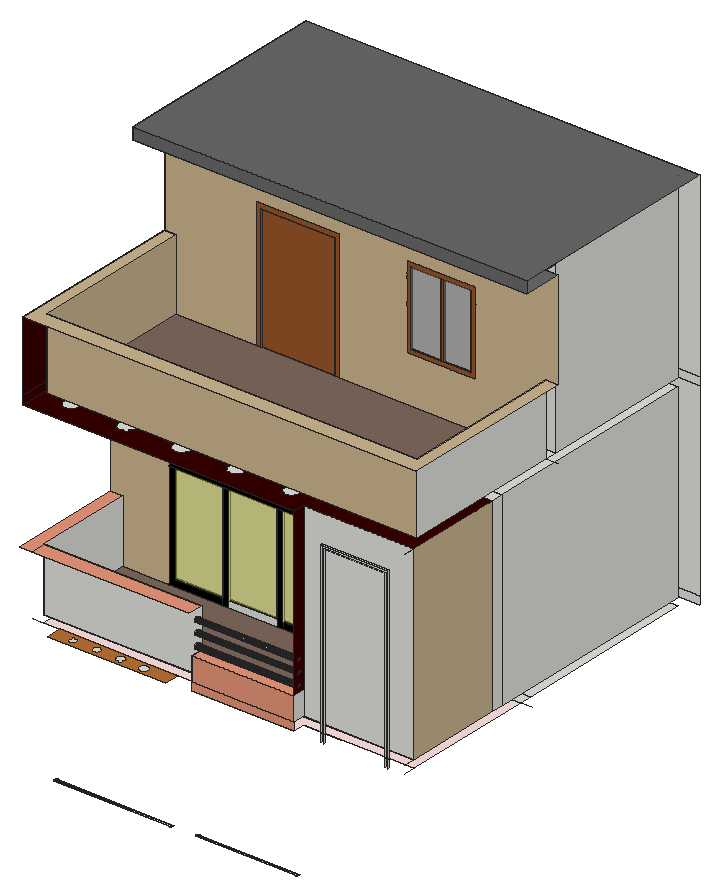
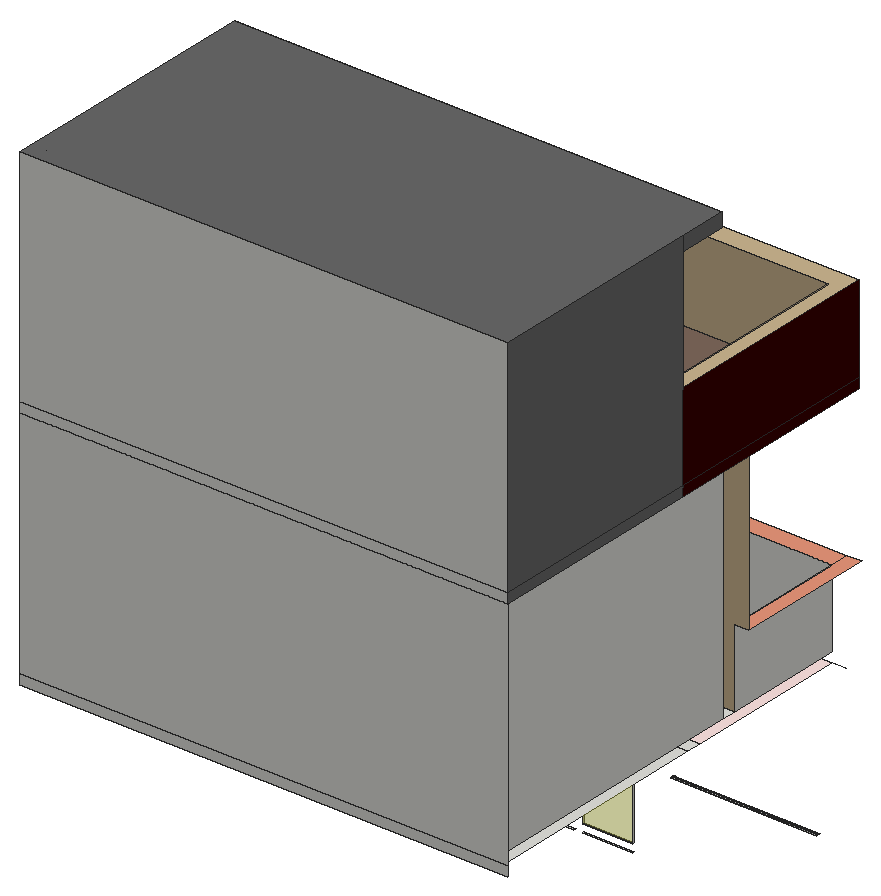
# SketchUp Ruby script. Lengths in inches.
U = 1.inch
M = Sketchup.active_model
def pt(a) = Geom::Point3d.new(a.map { |v| v * U })
def face(e, loops, mat)
  f = e.add_face(loops[0].map { |a| pt(a) })
  loops[1..].each { |l| e.add_face(l.map { |a| pt(a) }).erase! }
  f.material = f.back_material = mat if mat
  f
end
# faces: each face lists its corners as indices into pts; further lists are holes
def faces(e, pts, list, mat = nil) = list.each { |f| face(e, (f[0].is_a?(Array) ? f : [f]).map { |l| l.map { |i| pts[i] } }, mat) }
# xy, xz, yz: faces in a plane at the given z, y or x. An outline is a flat list of corners, or four numbers for a rectangle; further outlines are holes
def ring(l) = l.size == 4 ? [[l[0], l[1]], [l[2], l[1]], [l[2], l[3]], [l[0], l[3]]] : l.each_slice(2).to_a
def flat(e, list, mat, &to3) = list.each { |f| face(e, (f[0].is_a?(Array) ? f : [f]).map { |l| ring(l).map { |u, v| to3.(u, v) } }, mat) }
def xy(e, z, list, mat = nil) = flat(e, list, mat) { |x, y| [x, y, z] }
def xz(e, y, list, mat = nil) = flat(e, list, mat) { |x, z| [x, y, z] }
def yz(e, x, list, mat = nil) = flat(e, list, mat) { |y, z| [x, y, z] }
def lines(e, pts, list) = list.each { |a, b| e.add_line(pt(pts[a]), pt(pts[b])) }
# prism: a flat outline (further loops are holes) pulled along v
def prism(e, loops, v, mat = nil)
  f = face(e, loops, mat); d = Geom::Vector3d.new(v.map { |x| x * U })
  f.pushpull(f.normal.samedirection?(d) ? d.length : -d.length)
end
def box(e, o, s, mat = nil) = prism(e, [[o, [o[0] + s[0], o[1], o[2]], [o[0] + s[0], o[1] + s[1], o[2]], [o[0], o[1] + s[1], o[2]]]], [0, 0, s[2]], mat)
def at(x, y, z, deg = 0) = Geom::Transformation.translation(pt([x, y, z])) * Geom::Transformation.rotation(ORIGIN, Z_AXIS, deg.degrees)
def axes(o, x, y, z) = Geom::Transformation.new([*x, 0, *y, 0, *z, 0, *pt(o).to_a, 1])
def part(name) = M.definitions.add(name)
# library, detail: a bought-in or finely detailed component or shape, given as its bounding box
def library(name, o, s) = part(name).tap { |d| box(d.entities, o, s) }
def detail(e, o, s) = box(e.add_group.entities, o, s)
def put(e, d, t, mat = nil) = e.add_instance(d, t).tap { |i| i.material = mat if mat }
def group(e, t, mat = nil) = e.add_group.tap { |g| g.transformation = t; g.material = mat if mat }.entities
root = M.entities
M.materials.add("[0007_MistyRose]").color = [255, 228, 225]
M.materials.add("[0014_DarkSalmon]").color = [233, 150, 122]
M.materials.add("[0022_Maroon]").color = [56, 0, 0]
M.materials.add("[0032_Moccasin]").color = [204, 182, 144]
M.materials.add("[0134_DimGray]").color = [105, 105, 105]
M.materials.add("[0137_Black]").color = [0, 0, 0]
M.materials.add("[Granite Brown]").color = [126, 104, 91]
M.materials.add("[Translucent Glass Gray]").color = [220, 221, 73]
M.materials["[Translucent Glass Gray]"].alpha = 0.5
M.materials.add("[Translucent Glass Gray]1").color = [128, 128, 128]
M.materials["[Translucent Glass Gray]1"].alpha = 0.5
M.materials.add("[Wood Cherry Original]").color = [152, 86, 42]
M.materials.add("[Wood Floor Dark]").color = [186, 114, 51]
xy(root,776.75,[[98.58,227,160.58,229],[170.58,227,232.58,229],[242.58,227,307.71,229]])
xy(root,786.75,[[98.58,227,160.58,229],[170.58,227,232.58,229],[242.58,227,307.71,229]])
xy(root,854.9375,[[98.58,227,160.58,229],[170.58,227,232.58,229],[242.58,227,307.71,229]])
xy(root,856.52,[[370.68,227,426.27,229],[434.59,227,482.8,229]])
xy(root,924,[[71.83,5.5,70.28,5.7,68.83,6.3,67.59,7.26,66.63,8.5,66.03,9.95,65.83,11.5,66.03,13.05,66.63,14.5,67.59,15.74,68.83,16.7,70.28,17.3,71.83,17.5,73.38,17.3,74.83,16.7,76.07,15.74,77.02,14.5,77.625,13.05,77.83,11.5,77.625,9.95,77.02,8.5,76.07,7.26,74.83,6.3,73.38,5.7],[107.83,5.5,106.28,5.7,104.83,6.3,103.59,7.26,102.63,8.5,102.03,9.95,101.83,11.5,102.03,13.05,102.63,14.5,103.59,15.74,104.83,16.7,106.28,17.3,107.83,17.5,109.38,17.3,110.83,16.7,112.07,15.74,113.02,14.5,113.625,13.05,113.83,11.5,113.625,9.95,113.02,8.5,112.07,7.26,110.83,6.3,109.38,5.7],[143.83,5.5,142.28,5.7,140.83,6.3,139.59,7.26,138.63,8.5,138.03,9.95,137.83,11.5,138.03,13.05,138.63,14.5,139.59,15.74,140.83,16.7,142.28,17.3,143.83,17.5,145.38,17.3,146.83,16.7,148.07,15.74,149.02,14.5,149.625,13.05,149.83,11.5,149.625,9.95,149.02,8.5,148.07,7.26,146.83,6.3,145.38,5.7],[179.83,5.5,178.28,5.7,176.83,6.3,175.59,7.26,174.63,8.5,174.03,9.95,173.83,11.5,174.03,13.05,174.63,14.5,175.59,15.74,176.83,16.7,178.28,17.3,179.83,17.5,181.38,17.3,182.83,16.7,184.07,15.74,185.02,14.5,185.625,13.05,185.83,11.5,185.625,9.95,185.02,8.5,184.07,7.26,182.83,6.3,181.38,5.7],[18,227,582,245],
  [18,245,582,527]])
xy(root,924,[[258,5,258,23,18,23,18,227,582,227,582,23,414,23,414,5]],"[0007_MistyRose]")
xy(root,924,[[[42,0,222,23],[107.83,5.5,109.38,5.7,110.83,6.3,112.07,7.26,113.02,8.5,113.625,9.95,113.83,11.5,113.625,13.05,113.02,14.5,112.07,15.74,110.83,16.7,109.38,17.3,107.83,17.5,106.28,17.3,104.83,16.7,103.59,15.74,102.63,14.5,102.03,13.05,101.83,11.5,102.03,9.95,102.63,8.5,103.59,7.26,104.83,6.3,106.28,5.7],[143.83,5.5,145.38,5.7,146.83,6.3,148.07,7.26,149.02,8.5,149.625,9.95,149.83,11.5,149.625,13.05,149.02,14.5,148.07,15.74,146.83,16.7,145.38,17.3,143.83,17.5,142.28,17.3,140.83,16.7,139.59,15.74,138.63,14.5,138.03,13.05,137.83,11.5,138.03,9.95,138.63,8.5,139.59,7.26,140.83,6.3,142.28,5.7],[179.83,5.5,181.38,5.7,182.83,6.3,184.07,7.26,185.02,8.5,185.625,9.95,185.83,11.5,185.625,13.05,185.02,14.5,184.07,15.74,182.83,16.7,181.38,17.3,179.83,17.5,178.28,17.3,176.83,16.7,175.59,15.74,174.63,14.5,174.03,13.05,173.83,11.5,174.03,9.95,174.63,8.5,175.59,7.26,176.83,6.3,178.28,5.7],[71.83,5.5,73.38,5.7,74.83,6.3,76.07,7.26,77.02,8.5,77.625,9.95,77.83,11.5,77.625,13.05,77.02,14.5,76.07,15.74,74.83,16.7,73.38,17.3,71.83,17.5,70.28,17.3,68.83,16.7,67.59,15.74,66.63,14.5,66.03,13.05,65.83,11.5,66.03,9.95,66.63,8.5,67.59,7.26,68.83,6.3,70.28,5.7]]],"[Wood Floor Dark]")
xy(root,936,[[258,5,414,23],[18,173,582,191],[18,191,582,527]])
xy(root,936,[[18,23,582,173]],"[Granite Brown]")
xy(root,945.78,[[98.55,173,170.55,174],[180.55,173,252.55,174],[262.55,173,328.74,174]])
xy(root,972,[[258,5,414,23]],"[0014_DarkSalmon]")
xy(root,1032,[[0,0,18,173],[18,0,258,23]],"[0014_DarkSalmon]")
xy(root,1037.84,[[425.92,173,473.61,174],[479.91,173,525.8,174]])
xy(root,1097.25,[[98.55,173,170.55,174],[180.55,173,252.55,174],[262.55,173,328.74,174]])
xy(root,1107.25,[[98.55,173,170.55,174],[180.55,173,252.55,174],[262.55,173,328.74,174]])
xy(root,1169.47,[[98.55,173,170.55,174],[180.55,173,252.55,174],[262.55,173,328.74,174]])
xy(root,1171.97,[[425.92,173,473.61,174],[479.91,173,525.8,174]])
xy(root,1189.26,[[460.74,3,553.26,5]])
xy(root,1194.14,[[455.86,3,558.14,5]])
xy(root,1224,[[44.38,30.31,41.27,30.72,38.38,31.91,35.89,33.82,33.99,36.31,32.79,39.2,32.38,42.31,32.79,45.41,33.99,48.31,35.89,50.79,38.38,52.7,41.27,53.9,44.38,54.31,47.48,53.9,50.38,52.7,52.86,50.79,54.77,48.31,55.97,45.41,56.38,42.31,55.97,39.2,54.77,36.31,52.86,33.82,50.38,31.91,47.48,30.72],[128.38,30.31,125.27,30.72,122.38,31.91,119.89,33.82,117.99,36.31,116.79,39.2,116.38,42.31,116.79,45.41,117.99,48.31,119.89,50.79,122.38,52.7,125.27,53.9,128.38,54.31,131.48,53.9,134.38,52.7,136.86,50.79,138.77,48.31,139.97,45.41,140.38,42.31,139.97,39.2,138.77,36.31,136.86,33.82,134.38,31.91,131.48,30.72],[212.38,30.31,209.27,30.72,206.38,31.91,203.89,33.82,201.99,36.31,200.79,39.2,200.38,42.31,200.79,45.41,201.99,48.31,203.89,50.79,206.38,52.7,209.27,53.9,212.38,54.31,215.48,53.9,218.38,52.7,220.86,50.79,222.77,48.31,223.97,45.41,224.38,42.31,223.97,39.2,222.77,36.31,220.86,33.82,218.38,31.91,215.48,30.72],[296.38,30.31,293.27,30.72,290.38,31.91,287.89,33.82,285.99,36.31,284.79,39.2,284.38,42.31,284.79,45.41,285.99,48.31,287.89,50.79,290.38,52.7,293.27,53.9,296.38,54.31,299.48,53.9,302.38,52.7,304.86,50.79,306.77,48.31,307.97,45.41,308.38,42.31,307.97,39.2,306.77,36.31,304.86,33.82,302.38,31.91,299.48,30.72],[380.38,30.31,377.27,30.72,374.38,31.91,371.89,33.82,369.99,36.31,368.79,39.2,368.38,42.31,368.79,45.41,369.99,48.31,371.89,50.79,374.38,52.7,377.27,53.9,380.38,54.31,383.48,53.9,386.38,52.7,388.86,50.79,390.77,48.31,391.97,45.41,392.38,42.31,391.97,39.2,390.77,36.31,388.86,33.82,386.38,31.91,383.48,30.72],
  [18,173,582,191],[18,191,582,527]])
xy(root,1224,[[[0,5,0,173,582,173,582,23,414,23,414,5],[380.38,30.31,383.48,30.72,386.38,31.91,388.86,33.82,390.77,36.31,391.97,39.2,392.38,42.31,391.97,45.41,390.77,48.31,388.86,50.79,386.38,52.7,383.48,53.9,380.38,54.31,377.27,53.9,374.38,52.7,371.89,50.79,369.99,48.31,368.79,45.41,368.38,42.31,368.79,39.2,369.99,36.31,371.89,33.82,374.38,31.91,377.27,30.72],[296.38,30.31,299.48,30.72,302.38,31.91,304.86,33.82,306.77,36.31,307.97,39.2,308.38,42.31,307.97,45.41,306.77,48.31,304.86,50.79,302.38,52.7,299.48,53.9,296.38,54.31,293.27,53.9,290.38,52.7,287.89,50.79,285.99,48.31,284.79,45.41,284.38,42.31,284.79,39.2,285.99,36.31,287.89,33.82,290.38,31.91,293.27,30.72],[212.38,30.31,215.48,30.72,218.38,31.91,220.86,33.82,222.77,36.31,223.97,39.2,224.38,42.31,223.97,45.41,222.77,48.31,220.86,50.79,218.38,52.7,215.48,53.9,212.38,54.31,209.27,53.9,206.38,52.7,203.89,50.79,201.99,48.31,200.79,45.41,200.38,42.31,200.79,39.2,201.99,36.31,203.89,33.82,206.38,31.91,209.27,30.72],[128.38,30.31,131.48,30.72,134.38,31.91,136.86,33.82,138.77,36.31,139.97,39.2,140.38,42.31,139.97,45.41,138.77,48.31,136.86,50.79,134.38,52.7,131.48,53.9,128.38,54.31,125.27,53.9,122.38,52.7,119.89,50.79,117.99,48.31,116.79,45.41,116.38,42.31,116.79,39.2,117.99,36.31,119.89,33.82,122.38,31.91,125.27,30.72],[44.38,30.31,47.48,30.72,50.38,31.91,52.86,33.82,54.77,36.31,55.97,39.2,56.38,42.31,55.97,45.41,54.77,48.31,52.86,50.79,50.38,52.7,47.48,53.9,44.38,54.31,41.27,53.9,38.38,52.7,35.89,50.79,33.99,48.31,32.79,45.41,32.38,42.31,32.79,39.2,33.99,36.31,35.89,33.82,38.38,31.91,41.27,30.72]]],"[0022_Maroon]")
xy(root,1236,[[18,275,18,293,582,293,582,275,260.03,275,260.03,277,147.3125,277,147.3125,275],[18,293,582,527]])
xy(root,1236,[[18,29,582,29,582,275,260.03,275,260.03,277,147.3125,277,147.3125,275,18,275]],"[Granite Brown]")
xy(root,1312.99,[[376.41,275,421.71,277],[425.37,275,467,277]],"[0134_DimGray]")
xy(root,1344,[[0,5,600,5,600,275,582,275,582,29,18,29,18,275,0,275]],"[0032_Moccasin]")
xy(root,1425.14,[[147.3125,275,260.03,277]],"[0134_DimGray]")
xy(root,1425.83,[[376.41,275,421.71,277],[425.37,275,467,277]],"[0134_DimGray]")
xy(root,1494,[[18,293,582,527]])
xy(root,1494,[[0,215,600,275]],"[0134_DimGray]")
xy(root,1512,[[0,215,600,545]],"[0134_DimGray]")
xz(root,5,[[258,924,414,936],[258,936,414,972]],"[0014_DarkSalmon]")
xz(root,23,[[18,936,258,1032],[258,936,414,972],[414,936,582,1224]])
xz(root,29,[[18,1236,582,1344]],"[0032_Moccasin]")
xz(root,173,[[180.55,936,252.55,945.78]])
xz(root,173,[[[18,936,88.77,936,88.77,1179.25,338.52,1179.25,338.52,936,582,936,582,1224,0,1224,0,1032,18,1032],[418.65,1030.5625,533.08,1179.25]]],"[0032_Moccasin]")
xz(root,173,[[88.77,936,170.55,936,170.55,945.78,98.55,945.78,98.55,1097.25,88.77,1097.25],[170.55,936,180.55,1097.25],[252.55,936,262.55,1097.25],[262.55,936,338.52,936,338.52,1097.25,328.74,1097.25,328.74,945.78,262.55,945.78],[[418.65,1030.5625,533.08,1179.25],[425.92,1037.84,473.61,1171.97],[479.91,1037.84,525.8,1171.97]],
  [[88.77,1097.25,338.52,1179.25],[180.55,1107.25,252.55,1169.47],[98.55,1107.25,170.55,1169.47],[262.55,1107.25,328.74,1169.47]]],"[0137_Black]")
xz(root,174,[[98.55,945.78,170.55,1097.25],[180.55,945.78,252.55,1097.25],[262.55,945.78,328.74,1097.25],[425.92,1037.84,473.61,1171.97],[479.91,1037.84,525.8,1171.97],
  [98.55,1107.25,170.55,1169.47],[180.55,1107.25,252.55,1169.47],[262.55,1107.25,328.74,1169.47]],"[Translucent Glass Gray]")
xz(root,191,[[18,936,582,1224]])
xz(root,215,[[0,1494,600,1512]],"[0134_DimGray]")
xz(root,229,[[98.58,786.75,160.58,854.9375],[170.58,786.75,232.58,854.9375],[242.58,786.75,307.71,854.9375]],"[Translucent Glass Gray]")
xz(root,275,[[0,1236,18,1344]])
xz(root,275,[[[18,1236,139.2,1236,139.2,1433.25,268.14,1433.25,268.14,1236,582,1236,582,1344,600,1344,600,1494,0,1494,0,1344,18,1344],[368.99,1305.5625,474.42,1433.25]]],"[0032_Moccasin]")
xz(root,275,[[139.2,1236,147.3125,1236,147.3125,1425.14,260.03,1425.14,260.03,1236,268.14,1236,268.14,1433.25,139.2,1433.25],[[368.99,1305.5625,474.42,1433.25],[376.41,1312.99,467,1425.83]],[421.71,1312.99,425.37,1425.83]],"[Wood Cherry Original]")
xz(root,277,[[376.41,1312.99,421.71,1425.83],[425.37,1312.99,467,1425.83]],"[Translucent Glass Gray]1")
xz(root,277,[[147.3125,1236,260.03,1425.14]],"[Wood Cherry Original]")
xz(root,293,[[18,1236,582,1494]])
xz(root,527,[[18,936,582,1224],[18,1236,582,1494]])
xz(root,545,[[0,924,600,936],[0,936,600,1224],[0,1224,600,1236],[0,1236,600,1512]])
yz(root,0,[[5,1224,275,1236],[5,1236,275,1344]],"[0022_Maroon]")
yz(root,0,[[275,1224,545,1236],[275,1236,545,1512],[215,1494,275,1512]],"[0134_DimGray]")
yz(root,18,[[23,936,173,1032],[191,936,527,1224],[293,1236,527,1494]])
yz(root,18,[[29,1236,275,1344]],"[0032_Moccasin]")
yz(root,98.55,[[173,945.78,174,1097.25],[173,1107.25,174,1169.47]])
yz(root,98.58,[[227,786.75,229,854.9375]])
yz(root,147.3125,[[275,1236,277,1425.14]],"[0134_DimGray]")
yz(root,160.58,[[227,786.75,229,854.9375]])
yz(root,170.55,[[173,945.78,174,1097.25],[173,1107.25,174,1169.47]])
yz(root,170.58,[[227,786.75,229,854.9375]])
yz(root,180.55,[[173,945.78,174,1097.25],[173,1107.25,174,1169.47]])
yz(root,232.58,[[227,786.75,229,854.9375]])
yz(root,242.58,[[227,786.75,229,854.9375]])
yz(root,252.55,[[173,945.78,174,1097.25],[173,1107.25,174,1169.47]])
yz(root,258,[[5,936,23,972],[14,977.83,13.63,977.85,13.27,977.91,12.92,978,12.57,978.14,12.25,978.3,11.9375,978.5,11.65,978.73,11.39,978.99,11.16,979.28,10.96,979.59,10.8,979.91,10.66,980.26,10.57,980.61,10.51,980.97,10.49,981.34,10.51,981.71,10.57,982.07,10.66,982.42,10.8,982.77,10.96,983.09,11.16,983.4,11.39,983.6875,11.65,983.95,11.9375,984.18,12.25,984.38,12.57,984.54,12.92,984.68,13.27,984.77,13.63,984.83,14,984.85,14.37,984.83,14.73,984.77,15.08,984.68,15.43,984.54,15.75,984.38,16.0625,984.18,16.35,983.95,16.61,983.6875,16.84,983.4,17.04,983.09,17.2,982.77,17.34,982.42,17.43,982.07,17.49,981.71,17.51,981.34,17.49,980.97,17.43,980.61,17.34,980.26,17.2,979.91,17.04,979.59,16.84,979.28,16.61,978.99,16.35,978.73,16.0625,978.5,15.75,978.3,15.43,978.14,15.08,978,14.73,977.91,14.37,977.85],[14,996.07,13.66,996.09,13.32,996.14,12.99,996.23,12.67,996.35,12.36,996.51,12.08,996.69,11.81,996.91,11.57,997.15,11.35,997.42,11.17,997.7,11.01,998.01,10.89,998.33,10.8,998.66,10.75,999,10.73,999.34,10.75,999.68,10.8,1000.02,10.89,1000.35,11.01,1000.67,11.17,1000.98,11.35,1001.26,11.57,1001.53,11.81,1001.77,12.08,1001.99,12.36,1002.17,12.67,1002.33,12.99,1002.45,13.32,1002.54,13.66,1002.6,14,1002.61,14.34,1002.6,14.68,1002.54,15.01,1002.45,15.33,1002.33,15.64,1002.17,15.92,1001.99,16.19,1001.77,16.43,1001.53,16.65,1001.26,16.83,1000.98,16.99,1000.67,17.11,1000.35,17.2,1000.02,17.25,999.68,17.27,999.34,17.25,999,17.2,998.66,17.11,998.33,16.99,998.01,16.83,997.7,16.65,997.42,16.43,997.15,16.19,996.91,15.92,996.69,15.64,996.51,15.33,996.35,15.01,996.23,14.68,996.14,14.34,996.09],[14,1013.83,13.63,1013.85,13.27,1013.91,12.92,1014.01,12.57,1014.14,12.25,1014.3,11.9375,1014.5,11.65,1014.74,11.39,1014.99,11.16,1015.28,10.96,1015.59,10.8,1015.91,10.67,1016.26,10.57,1016.61,10.51,1016.97,10.49,1017.34,10.51,1017.71,10.57,1018.07,10.67,1018.42,10.8,1018.77,10.96,1019.09,11.16,1019.4,11.39,1019.6875,11.65,1019.95,11.9375,1020.18,12.25,1020.375,12.57,1020.54,12.92,1020.68,13.27,1020.77,13.63,1020.83,14,1020.85,14.37,1020.83,14.73,1020.77,15.08,1020.68,15.43,1020.54,15.75,1020.375,16.0625,1020.18,16.35,1019.95,16.61,1019.6875,16.84,1019.4,17.04,1019.09,17.2,1018.77,17.33,1018.42,17.43,1018.07,17.49,1017.71,17.51,1017.34,17.49,1016.97,17.43,1016.61,17.33,1016.26,17.2,1015.91,17.04,1015.59,16.84,1015.28,16.61,1014.99,16.35,1014.74,16.0625,1014.5,15.75,1014.3,15.43,1014.14,15.08,1014.01,14.73,1013.91,14.37,1013.85]])
yz(root,260.03,[[275,1236,277,1425.14]],"[0134_DimGray]")
yz(root,262.55,[[173,945.78,174,1097.25],[173,1107.25,174,1169.47]])
yz(root,307.71,[[227,786.75,229,854.9375]])
yz(root,328.74,[[173,945.78,174,1097.25],[173,1107.25,174,1169.47]])
yz(root,376.41,[[275,1312.99,277,1425.83]],"[0134_DimGray]")
yz(root,414,[[5,936,23,972]])
yz(root,414,[[[5,972,23,1224],[14,977.83,14.37,977.85,14.73,977.91,15.08,978,15.43,978.14,15.75,978.3,16.0625,978.5,16.35,978.73,16.61,978.99,16.84,979.28,17.04,979.59,17.2,979.91,17.34,980.26,17.43,980.61,17.49,980.97,17.51,981.34,17.49,981.71,17.43,982.07,17.34,982.42,17.2,982.77,17.04,983.09,16.84,983.4,16.61,983.6875,16.35,983.95,16.0625,984.18,15.75,984.38,15.43,984.54,15.08,984.68,14.73,984.77,14.37,984.83,14,984.85,13.63,984.83,13.27,984.77,12.92,984.68,12.57,984.54,12.25,984.38,11.9375,984.18,11.65,983.95,11.39,983.6875,11.16,983.4,10.96,983.09,10.8,982.77,10.66,982.42,10.57,982.07,10.51,981.71,10.49,981.34,10.51,980.97,10.57,980.61,10.66,980.26,10.8,979.91,10.96,979.59,11.16,979.28,11.39,978.99,11.65,978.73,11.9375,978.5,12.25,978.3,12.57,978.14,12.92,978,13.27,977.91,13.63,977.85],[14,1013.83,14.37,1013.85,14.73,1013.91,15.08,1014.01,15.43,1014.14,15.75,1014.3,16.0625,1014.5,16.35,1014.74,16.61,1014.99,16.84,1015.28,17.04,1015.59,17.2,1015.91,17.33,1016.26,17.43,1016.61,17.49,1016.97,17.51,1017.34,17.49,1017.71,17.43,1018.07,17.33,1018.42,17.2,1018.77,17.04,1019.09,16.84,1019.4,16.61,1019.6875,16.35,1019.95,16.0625,1020.18,15.75,1020.375,15.43,1020.54,15.08,1020.68,14.73,1020.77,14.37,1020.83,14,1020.85,13.63,1020.83,13.27,1020.77,12.92,1020.68,12.57,1020.54,12.25,1020.375,11.9375,1020.18,11.65,1019.95,11.39,1019.6875,11.16,1019.4,10.96,1019.09,10.8,1018.77,10.67,1018.42,10.57,1018.07,10.51,1017.71,10.49,1017.34,10.51,1016.97,10.57,1016.61,10.67,1016.26,10.8,1015.91,10.96,1015.59,11.16,1015.28,11.39,1014.99,11.65,1014.74,11.9375,1014.5,12.25,1014.3,12.57,1014.14,12.92,1014.01,13.27,1013.91,13.63,1013.85],[14,996.07,14.34,996.09,14.68,996.14,15.01,996.23,15.33,996.35,15.64,996.51,15.92,996.69,16.19,996.91,16.43,997.15,16.65,997.42,16.83,997.7,16.99,998.01,17.11,998.33,17.2,998.66,17.25,999,17.27,999.34,17.25,999.68,17.2,1000.02,17.11,1000.35,16.99,1000.67,16.83,1000.98,16.65,1001.26,16.43,1001.53,16.19,1001.77,15.92,1001.99,15.64,1002.17,15.33,1002.33,15.01,1002.45,14.68,1002.54,14.34,1002.6,14,1002.61,13.66,1002.6,13.32,1002.54,12.99,1002.45,12.67,1002.33,12.36,1002.17,12.08,1001.99,11.81,1001.77,11.57,1001.53,11.35,1001.26,11.17,1000.98,11.01,1000.67,10.89,1000.35,10.8,1000.02,10.75,999.68,10.73,999.34,10.75,999,10.8,998.66,10.89,998.33,11.01,998.01,11.17,997.7,11.35,997.42,11.57,997.15,11.81,996.91,12.08,996.69,12.36,996.51,12.67,996.35,12.99,996.23,13.32,996.14,13.66,996.09]]],"[0022_Maroon]")
yz(root,421.71,[[275,1312.99,277,1425.83]],"[0134_DimGray]")
yz(root,425.37,[[275,1312.99,277,1425.83]],"[0134_DimGray]")
yz(root,425.92,[[173,1037.84,174,1171.97]])
yz(root,455.86,[[3,924,5,936],[3,936,5,1194.14]])
yz(root,460.74,[[3,924,5,936],[3,936,5,1189.26]])
yz(root,467,[[275,1312.99,277,1425.83]],"[0134_DimGray]")
yz(root,473.61,[[173,1037.84,174,1171.97]])
yz(root,479.91,[[173,1037.84,174,1171.97]])
yz(root,525.8,[[173,1037.84,174,1171.97]])
yz(root,553.26,[[3,924,5,936],[3,936,5,1189.26]])
yz(root,558.14,[[3,924,5,936],[3,936,5,1194.14]])
yz(root,582,[[173,936,191,1224],[191,936,527,1224],[29,1236,275,1344],[293,1236,527,1494]])
yz(root,582,[[23,936,173,1224]],"[0032_Moccasin]")
p = [[42,12.5,722.6],[42,11.88,722.12],[222,11.88,722.12],[222,12.5,722.6],[258,12.5,722.6],[258,11.88,722.12],
  [414,11.88,722.12],[414,12.5,722.6],[42,16.12,722.12],[42,15.5,722.6],[222,15.5,722.6],[222,16.12,722.12],
  [258,16.12,722.12],[258,15.5,722.6],[414,15.5,722.6],[414,16.12,722.12],[42,13.22,722.9],[222,13.22,722.9],
  [258,13.22,722.9],[414,13.22,722.9],[42,14.78,722.9],[222,14.78,722.9],[258,14.78,722.9],[414,14.78,722.9],
  [42,14,723],[222,14,723],[258,14,723],[414,14,723],[258,13.63,977.85],[258,14,977.83],
  [414,14,977.83],[414,13.63,977.85],[258,14.37,977.85],[414,14.37,977.85],[258,12.92,978],[258,13.27,977.91],
  [414,13.27,977.91],[414,12.92,978],[258,14.73,977.91],[414,14.73,977.91],[258,15.08,978],[414,15.08,978],
  [258,12.57,978.14],[414,12.57,978.14],[258,15.43,978.14],[414,15.43,978.14],[258,12.25,978.3],[414,12.25,978.3],
  [258,15.75,978.3],[414,15.75,978.3],[258,11.9375,978.5],[414,11.9375,978.5],[258,16.0625,978.5],[414,16.0625,978.5],
  [258,11.65,978.73],[414,11.65,978.73],[258,16.35,978.73],[414,16.35,978.73],[258,11.39,978.99],[414,11.39,978.99],
  [258,16.61,978.99],[414,16.61,978.99],[258,11.16,979.28],[414,11.16,979.28],[258,16.84,979.28],[414,16.84,979.28],
  [258,10.96,979.59],[414,10.96,979.59],[258,17.04,979.59],[414,17.04,979.59],[258,10.8,979.91],[414,10.8,979.91],
  [258,17.2,979.91],[414,17.2,979.91],[258,10.66,980.26],[414,10.66,980.26],[258,17.34,980.26],[414,17.34,980.26],
  [258,10.57,980.61],[414,10.57,980.61],[258,17.43,980.61],[414,17.43,980.61],[258,10.51,980.97],[414,10.51,980.97],
  [258,17.49,980.97],[414,17.49,980.97],[258,10.49,981.34],[414,10.49,981.34],[258,17.51,981.34],[414,17.51,981.34],
  [258,10.51,981.71],[414,10.51,981.71],[258,17.49,981.71],[414,17.49,981.71],[258,10.57,982.07],[414,10.57,982.07],
  [258,17.43,982.07],[414,17.43,982.07],[258,10.66,982.42],[414,10.66,982.42],[258,17.34,982.42],[414,17.34,982.42],
  [258,10.8,982.77],[414,10.8,982.77],[258,17.2,982.77],[414,17.2,982.77],[258,10.96,983.09],[414,10.96,983.09],
  [258,17.04,983.09],[414,17.04,983.09],[258,11.16,983.4],[414,11.16,983.4],[258,16.84,983.4],[414,16.84,983.4],
  [258,11.39,983.6875],[414,11.39,983.6875],[258,16.61,983.6875],[414,16.61,983.6875],[258,11.65,983.95],[414,11.65,983.95],
  [258,16.35,983.95],[414,16.35,983.95],[258,11.9375,984.18],[414,11.9375,984.18],[258,16.0625,984.18],[414,16.0625,984.18],
  [258,12.25,984.38],[414,12.25,984.38],[258,15.75,984.38],[414,15.75,984.38],[258,12.57,984.54],[414,12.57,984.54],
  [258,15.43,984.54],[414,15.43,984.54],[258,12.92,984.68],[414,12.92,984.68],[258,15.08,984.68],[414,15.08,984.68],
  [258,13.27,984.77],[414,13.27,984.77],[258,14.73,984.77],[414,14.73,984.77],[258,13.63,984.83],[414,13.63,984.83],
  [258,14,984.85],[414,14,984.85],[258,14.37,984.83],[414,14.37,984.83],[258,12.99,996.23],[258,13.32,996.14],
  [414,13.32,996.14],[414,12.99,996.23],[258,13.66,996.09],[414,13.66,996.09],[258,14,996.07],[414,14,996.07],
  [258,14.34,996.09],[414,14.34,996.09],[258,14.68,996.14],[414,14.68,996.14],[258,15.01,996.23],[414,15.01,996.23],
  [258,12.67,996.35],[414,12.67,996.35],[258,15.33,996.35],[414,15.33,996.35],[258,12.36,996.51],[414,12.36,996.51],
  [258,15.64,996.51],[414,15.64,996.51],[258,12.08,996.69],[414,12.08,996.69],[258,15.92,996.69],[414,15.92,996.69],
  [258,11.81,996.91],[414,11.81,996.91],[258,16.19,996.91],[414,16.19,996.91],[258,11.57,997.15],[414,11.57,997.15],
  [258,16.43,997.15],[414,16.43,997.15],[258,11.35,997.42],[414,11.35,997.42],[258,16.65,997.42],[414,16.65,997.42],
  [258,11.17,997.7],[414,11.17,997.7],[258,16.83,997.7],[414,16.83,997.7],[258,11.01,998.01],[414,11.01,998.01],
  [258,16.99,998.01],[414,16.99,998.01],[258,10.89,998.33],[414,10.89,998.33],[258,17.11,998.33],[414,17.11,998.33],
  [258,10.8,998.66],[414,10.8,998.66],[258,17.2,998.66],[414,17.2,998.66],[258,10.75,999],[414,10.75,999],
  [258,17.25,999],[414,17.25,999],[258,10.73,999.34],[414,10.73,999.34],[258,17.27,999.34],[414,17.27,999.34],
  [258,10.75,999.68],[414,10.75,999.68],[258,17.25,999.68],[414,17.25,999.68],[258,10.8,1000.02],[414,10.8,1000.02],
  [258,17.2,1000.02],[414,17.2,1000.02],[258,10.89,1000.35],[414,10.89,1000.35],[258,17.11,1000.35],[414,17.11,1000.35],
  [258,11.01,1000.67],[414,11.01,1000.67],[258,16.99,1000.67],[414,16.99,1000.67],[258,11.17,1000.98],[414,11.17,1000.98],
  [258,16.83,1000.98],[414,16.83,1000.98],[258,11.35,1001.26],[414,11.35,1001.26],[258,16.65,1001.26],[414,16.65,1001.26],
  [258,11.57,1001.53],[414,11.57,1001.53],[258,16.43,1001.53],[414,16.43,1001.53],[258,11.81,1001.77],[414,11.81,1001.77],
  [258,16.19,1001.77],[414,16.19,1001.77],[258,12.08,1001.99],[414,12.08,1001.99],[258,15.92,1001.99],[414,15.92,1001.99],
  [258,12.36,1002.17],[414,12.36,1002.17],[258,15.64,1002.17],[414,15.64,1002.17],[258,12.67,1002.33],[414,12.67,1002.33],
  [258,15.33,1002.33],[414,15.33,1002.33],[258,12.99,1002.45],[414,12.99,1002.45],[258,15.01,1002.45],[414,15.01,1002.45],
  [258,13.32,1002.54],[414,13.32,1002.54],[258,13.66,1002.6],[414,13.66,1002.6],[258,14.68,1002.54],[258,14.34,1002.6],
  [414,14.34,1002.6],[414,14.68,1002.54],[258,14,1002.61],[414,14,1002.61],[258,13.63,1013.85],[258,14,1013.83],
  [414,14,1013.83],[414,13.63,1013.85],[258,14.37,1013.85],[414,14.37,1013.85],[258,12.92,1014.01],[258,13.27,1013.91],
  [414,13.27,1013.91],[414,12.92,1014.01],[258,14.73,1013.91],[414,14.73,1013.91],[258,15.08,1014.01],[414,15.08,1014.01],
  [258,12.57,1014.14],[414,12.57,1014.14],[258,15.43,1014.14],[414,15.43,1014.14],[258,12.25,1014.3],[414,12.25,1014.3],
  [258,15.75,1014.3],[414,15.75,1014.3],[258,11.9375,1014.5],[414,11.9375,1014.5],[258,16.0625,1014.5],[414,16.0625,1014.5],
  [258,11.65,1014.74],[414,11.65,1014.74],[258,16.35,1014.74],[414,16.35,1014.74],[258,11.39,1014.99],[414,11.39,1014.99],
  [258,16.61,1014.99],[414,16.61,1014.99],[258,11.16,1015.28],[414,11.16,1015.28],[258,16.84,1015.28],[414,16.84,1015.28],
  [258,10.96,1015.59],[414,10.96,1015.59],[258,17.04,1015.59],[414,17.04,1015.59],[258,10.8,1015.91],[414,10.8,1015.91],
  [258,17.2,1015.91],[414,17.2,1015.91],[258,10.67,1016.26],[414,10.67,1016.26],[258,17.33,1016.26],[414,17.33,1016.26],
  [258,10.57,1016.61],[414,10.57,1016.61],[258,17.43,1016.61],[414,17.43,1016.61],[258,10.51,1016.97],[414,10.51,1016.97],
  [258,17.49,1016.97],[414,17.49,1016.97],[258,10.49,1017.34],[414,10.49,1017.34],[258,17.51,1017.34],[414,17.51,1017.34],
  [258,10.51,1017.71],[414,10.51,1017.71],[258,17.49,1017.71],[414,17.49,1017.71],[258,10.57,1018.07],[414,10.57,1018.07],
  [258,17.43,1018.07],[414,17.43,1018.07],[258,10.67,1018.42],[414,10.67,1018.42],[258,17.33,1018.42],[414,17.33,1018.42],
  [258,10.8,1018.77],[414,10.8,1018.77],[258,17.2,1018.77],[414,17.2,1018.77],[258,10.96,1019.09],[414,10.96,1019.09],
  [258,17.04,1019.09],[414,17.04,1019.09],[258,11.16,1019.4],[414,11.16,1019.4],[258,16.84,1019.4],[414,16.84,1019.4],
  [258,11.39,1019.6875],[414,11.39,1019.6875],[258,16.61,1019.6875],[414,16.61,1019.6875],[258,11.65,1019.95],[414,11.65,1019.95],
  [258,16.35,1019.95],[414,16.35,1019.95],[258,11.9375,1020.18],[414,11.9375,1020.18],[258,16.0625,1020.18],[414,16.0625,1020.18],
  [258,12.25,1020.375],[414,12.25,1020.375],[258,15.75,1020.375],[414,15.75,1020.375],[258,12.57,1020.54],[414,12.57,1020.54],
  [258,15.43,1020.54],[414,15.43,1020.54],[258,12.92,1020.68],[414,12.92,1020.68],[258,15.08,1020.68],[414,15.08,1020.68],
  [258,13.27,1020.77],[414,13.27,1020.77],[258,14.73,1020.77],[414,14.73,1020.77],[258,13.63,1020.83],[414,13.63,1020.83],
  [258,14,1020.85],[414,14,1020.85],[258,14.37,1020.83],[414,14.37,1020.83],[582,227,924],[600,227,924],
  [582,275,1236],[600,275,1236],[582,527,1494],[582,527,1512],[18,293,1494],[18,275,1494],
  [582,293,1494],[582,275,1494],[582,23,936],[582,5,936],[582,23,924],[582,5,924],
  [582,23,1224],[582,5,1224],[18,23,924],[0,23,924],[258,14,981.34],[414,14,981.34],
  [258,14,999.34],[414,14,999.34],[258,14,1017.34],[414,14,1017.34]]
faces(root,p,[[0,1,2,3],[4,5,6,7],[8,9,10,11],[12,13,14,15],[16,0,3,17],[18,4,7,19],[9,20,21,10],[13,22,23,14],
  [24,16,17,25],[26,18,19,27],[20,24,25,21],[22,26,27,23],[28,29,30,31],[29,32,33,30],[34,35,36,37],[35,28,31,36],
  [32,38,39,33],[38,40,41,39],[42,34,37,43],[40,44,45,41],[46,42,43,47],[44,48,49,45],[50,46,47,51],[48,52,53,49],
  [54,50,51,55],[52,56,57,53],[58,54,55,59],[56,60,61,57],[62,58,59,63],[60,64,65,61],[66,62,63,67],[64,68,69,65],
  [70,66,67,71],[68,72,73,69],[74,70,71,75],[72,76,77,73],[78,74,75,79],[76,80,81,77],[82,78,79,83],[80,84,85,81],
  [86,82,83,87],[84,88,89,85],[90,86,87,91],[88,92,93,89],[94,90,91,95],[92,96,97,93],[98,94,95,99],[96,100,101,97],
  [102,98,99,103],[100,104,105,101],[106,102,103,107],[104,108,109,105],[110,106,107,111],[108,112,113,109],[114,110,111,115],[112,116,117,113],
  [118,114,115,119],[116,120,121,117],[122,118,119,123],[120,124,125,121],[126,122,123,127],[124,128,129,125],[130,126,127,131],[128,132,133,129],
  [134,130,131,135],[132,136,137,133],[138,134,135,139],[136,140,141,137],[142,138,139,143],[144,142,143,145],[146,144,145,147],[140,146,147,141],
  [148,149,150,151],[149,152,153,150],[152,154,155,153],[154,156,157,155],[156,158,159,157],[158,160,161,159],[162,148,151,163],[160,164,165,161],
  [166,162,163,167],[164,168,169,165],[170,166,167,171],[168,172,173,169],[174,170,171,175],[172,176,177,173],[178,174,175,179],[176,180,181,177],
  [182,178,179,183],[180,184,185,181],[186,182,183,187],[184,188,189,185],[190,186,187,191],[188,192,193,189],[194,190,191,195],[192,196,197,193],
  [198,194,195,199],[196,200,201,197],[202,198,199,203],[200,204,205,201],[206,202,203,207],[204,208,209,205],[210,206,207,211],[208,212,213,209],
  [214,210,211,215],[212,216,217,213],[218,214,215,219],[216,220,221,217],[222,218,219,223],[220,224,225,221],[226,222,223,227],[224,228,229,225],
  [230,226,227,231],[228,232,233,229],[234,230,231,235],[232,236,237,233],[238,234,235,239],[236,240,241,237],[242,238,239,243],[240,244,245,241],
  [246,242,243,247],[244,248,249,245],[250,246,247,251],[248,252,253,249],[254,250,251,255],[252,256,257,253],[258,254,255,259],[260,258,259,261],
  [262,263,264,265],[256,262,265,257],[266,260,261,267],[263,266,267,264],[268,269,270,271],[269,272,273,270],[274,275,276,277],[275,268,271,276],
  [272,278,279,273],[278,280,281,279],[282,274,277,283],[280,284,285,281],[286,282,283,287],[284,288,289,285],[290,286,287,291],[288,292,293,289],
  [294,290,291,295],[292,296,297,293],[298,294,295,299],[296,300,301,297],[302,298,299,303],[300,304,305,301],[306,302,303,307],[304,308,309,305],
  [310,306,307,311],[308,312,313,309],[314,310,311,315],[312,316,317,313],[318,314,315,319],[316,320,321,317],[322,318,319,323],[320,324,325,321],
  [326,322,323,327],[324,328,329,325],[330,326,327,331],[328,332,333,329],[334,330,331,335],[332,336,337,333],[338,334,335,339],[336,340,341,337],
  [342,338,339,343],[340,344,345,341],[346,342,343,347],[344,348,349,345],[350,346,347,351],[348,352,353,349],[354,350,351,355],[352,356,357,353],
  [358,354,355,359],[356,360,361,357],[362,358,359,363],[360,364,365,361],[366,362,363,367],[364,368,369,365],[370,366,367,371],[368,372,373,369],
  [374,370,371,375],[372,376,377,373],[378,374,375,379],[376,380,381,377],[382,378,379,383],[384,382,383,385],[386,384,385,387],[380,386,387,381]])
lines(root,p,[[388,389],[390,391],[392,393],[394,395],[396,397],[398,399],[400,401],[402,403],[404,405],[406,407],[408,409],[410,411]])
